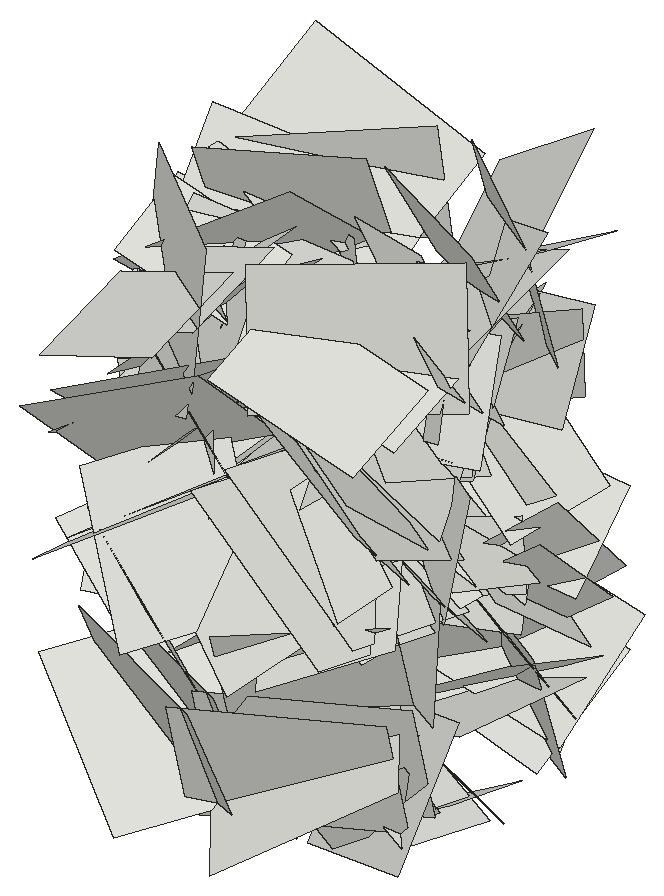
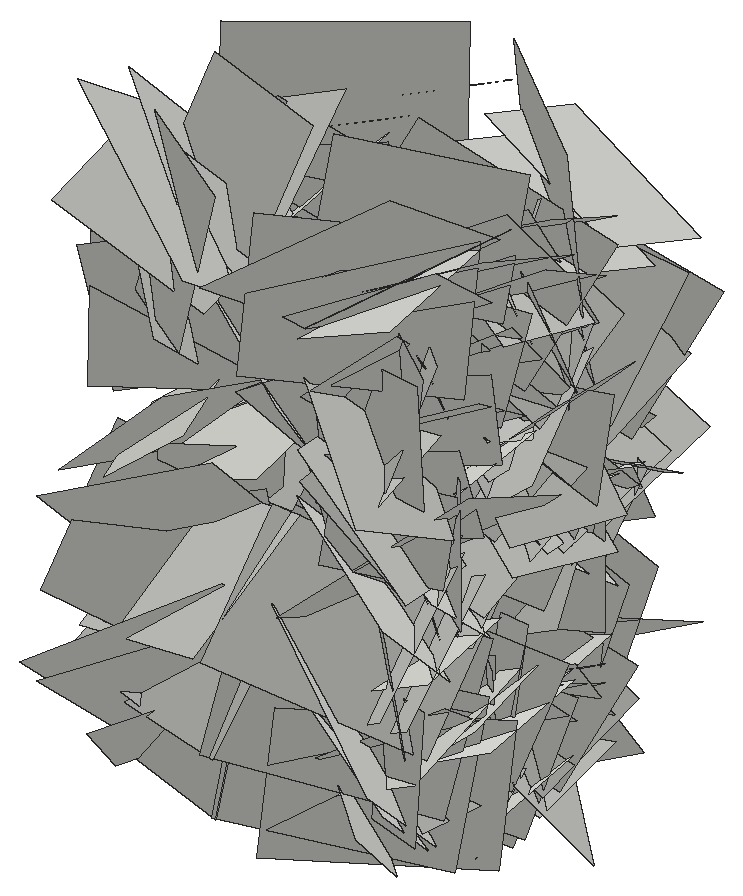
# SketchUp Ruby script. Lengths in inches.
U = 1.inch
M = Sketchup.active_model
def pt(a) = Geom::Point3d.new(a.map { |v| v * U })
def face(e, loops, mat)
  f = e.add_face(loops[0].map { |a| pt(a) })
  loops[1..].each { |l| e.add_face(l.map { |a| pt(a) }).erase! }
  f.material = f.back_material = mat if mat
  f
end
# faces: each face lists its corners as indices into pts; further lists are holes
def faces(e, pts, list, mat = nil) = list.each { |f| face(e, (f[0].is_a?(Array) ? f : [f]).map { |l| l.map { |i| pts[i] } }, mat) }
# xy, xz, yz: faces in a plane at the given z, y or x. An outline is a flat list of corners, or four numbers for a rectangle; further outlines are holes
def ring(l) = l.size == 4 ? [[l[0], l[1]], [l[2], l[1]], [l[2], l[3]], [l[0], l[3]]] : l.each_slice(2).to_a
def flat(e, list, mat, &to3) = list.each { |f| face(e, (f[0].is_a?(Array) ? f : [f]).map { |l| ring(l).map { |u, v| to3.(u, v) } }, mat) }
def xy(e, z, list, mat = nil) = flat(e, list, mat) { |x, y| [x, y, z] }
def xz(e, y, list, mat = nil) = flat(e, list, mat) { |x, z| [x, y, z] }
def yz(e, x, list, mat = nil) = flat(e, list, mat) { |y, z| [x, y, z] }
def lines(e, pts, list) = list.each { |a, b| e.add_line(pt(pts[a]), pt(pts[b])) }
# prism: a flat outline (further loops are holes) pulled along v
def prism(e, loops, v, mat = nil)
  f = face(e, loops, mat); d = Geom::Vector3d.new(v.map { |x| x * U })
  f.pushpull(f.normal.samedirection?(d) ? d.length : -d.length)
end
def box(e, o, s, mat = nil) = prism(e, [[o, [o[0] + s[0], o[1], o[2]], [o[0] + s[0], o[1] + s[1], o[2]], [o[0], o[1] + s[1], o[2]]]], [0, 0, s[2]], mat)
def at(x, y, z, deg = 0) = Geom::Transformation.translation(pt([x, y, z])) * Geom::Transformation.rotation(ORIGIN, Z_AXIS, deg.degrees)
def axes(o, x, y, z) = Geom::Transformation.new([*x, 0, *y, 0, *z, 0, *pt(o).to_a, 1])
def part(name) = M.definitions.add(name)
# library, detail: a bought-in or finely detailed component or shape, given as its bounding box
def library(name, o, s) = part(name).tap { |d| box(d.entities, o, s) }
def detail(e, o, s) = box(e.add_group.entities, o, s)
def put(e, d, t, mat = nil) = e.add_instance(d, t).tap { |i| i.material = mat if mat }
def group(e, t, mat = nil) = e.add_group.tap { |g| g.transformation = t; g.material = mat if mat }.entities
root = M.entities
c1 = part("Component\#6")
p = [[0.01,0,0],[0,3.24,4.54],[4.32,3.24,4.54],[4.33,0,0]]
faces(c1.entities,p,[[0,1,2,3]])
put(root,c1,axes([410.71,132.67,11.61],[-0.16439,-1.14375,-0.17253],[-0.24163,-0.14044,1.13591],[1.20204,-0.18465,0.20475]))
put(root,c1,axes([414.68,132.67,11.61],[0.16439,-1.14375,-0.17253],[0.24163,-0.14044,1.13591],[-1.20204,-0.18465,0.20475]))
put(root,c1,axes([410.71,126.24,11.02],[0.17433,0.41563,0.4957],[0.04437,0.50356,-0.43611],[0.68427,-0.13854,-0.09801]))
put(root,c1,axes([414.68,133.51,8.98],[0.15319,0.47062,-0.90401],[0.09722,-0.91536,-0.46187],[-1.07594,-0.0157,-0.17044]))
put(root,c1,axes([410.71,136.01,11.51],[0.06598,-0.27091,0.62957],[0.16839,0.62065,0.25136],[0.70672,-0.12259,-0.11867]))
put(root,c1,axes([410.71,130.2,1.79],[-0.1042,-0.77086,0.73803],[-0.17604,0.74317,0.75412],[1.11745,0.04519,0.18762]))
put(root,c1,axes([410.71,137.27,19.36],[-0.1763,0.15017,-0.9005],[0.15684,-0.89878,-0.17721],[0.95491,0.17535,-0.13715]))
put(root,c1,axes([414.68,136.42,13.64],[-0.14309,-0.55174,0.41683],[0.03038,0.41987,0.56505],[-0.73236,0.12522,-0.058]))
put(root,c1,axes([414.68,135.65,2.32],[0.1935,-1.06071,0.09437],[0.13048,0.11613,1.0671],[-1.12123,-0.16954,0.14047]))
put(root,c1,axes([410.71,132.96,18.89],[-0.10145,-0.91774,-0.17179],[0.02227,-0.17476,0.92192],[0.98945,-0.09016,-0.03837]))
put(root,c1,axes([410.71,133.07,14.74],[-0.12706,0.28525,0.91315],[0.02767,0.92092,-0.28425],[1.01369,0.01061,0.12222]))
put(root,c1,axes([410.71,135.14,15.06],[-0.15738,0.18416,-1.10832],[-0.16264,-1.1108,-0.16402],[1.17977,-0.12857,-0.17046]))
put(root,c1,axes([414.68,130.01,4.69],[-0.05447,0.12092,0.77662],[0.06993,0.77619,-0.11649],[-0.83019,0.05744,-0.06077]))
put(root,c1,axes([410.71,131.35,15.19],[0.02447,0.82058,-0.14823],[0.01236,-0.14859,-0.82075],[0.8838,-0.02064,0.01558]))
put(root,c1,axes([410.71,133.58,20.74],[-0.06025,0.71815,0.57437],[-0.00066,0.57544,-0.71955],[0.97476,0.04478,0.03501]))
put(root,c1,axes([410.71,133.14,16.06],[-0.03738,-0.31853,0.81486],[0.04959,0.81367,0.32009],[0.92608,-0.05642,0.01575]))
put(root,c1,axes([414.68,137.37,4.77],[0.01509,-0.67708,-0.46908],[0.05072,-0.46768,0.67651],[-0.87164,-0.03894,0.03124]))
put(root,c1,axes([410.71,128.53,16.93],[-0.30517,1.08519,-0.55956],[-0.1011,-0.59314,-1.10124],[1.29027,0.21019,-0.21864]))
put(root,c1,axes([410.71,127.92,4.7],[0.092,0.70183,0.2556],[0.07294,0.24871,-0.70628],[0.78837,-0.10491,0.03552]))
put(root,c1,axes([410.71,125.93,11.7],[0.16945,0.67455,-0.05214],[0.09647,-0.07453,-0.68517],[0.71064,-0.15073,0.10544]))
put(root,c1,axes([414.68,136.82,15.87],[0.16772,-0.74319,-0.48228],[-0.03783,-0.49486,0.75087],[-0.93836,-0.11289,-0.11647]))
put(root,c1,axes([414.68,131.86,3.01],[-0.01467,-0.55248,-0.51034],[0.00827,-0.51051,0.55244],[-0.7972,0.00487,0.01512]))
put(root,c1,axes([414.68,125.86,8.82],[-0.02658,0.53015,0.39509],[-0.11889,0.38623,-0.52538],[-0.69069,-0.08688,0.07523]))
put(root,c1,axes([410.71,127.95,5.4],[0.05879,0.74539,0.22064],[0.10629,0.21249,-0.74307],[0.81711,-0.08127,0.08079]))
put(root,c1,axes([414.68,131.99,-0.9375],[-0.0225,-0.54484,0.50649],[0.02225,0.50605,0.54525],[-0.78821,0.02984,0.00093]))
put(root,c1,axes([410.71,136.53,11.26],[-0.01536,-0.64622,-0.54667],[0.11065,-0.54394,0.64022],[0.89037,0.05645,-0.089]))
put(root,c1,axes([414.68,133.96,6.46],[0.0893,0.11056,0.97068],[0.19494,0.95507,-0.12474],[-1.01706,0.19277,0.06132]))
put(root,c1,axes([414.68,133.42,16.97],[0.14677,0.94615,0.46149],[0.22557,0.4307,-0.94687],[-1.09283,0.21597,-0.13346]))
put(root,c1,axes([410.71,127.34,21.1],[-0.03089,0.79811,0.32897],[0.11706,0.3299,-0.79059],[0.90753,-0.01539,0.11317]))
put(root,c1,axes([410.71,127.86,19.19],[-0.25173,1.01088,0.57921],[-0.04385,0.58343,-1.03521],[1.23418,0.22691,0.08136]))
put(root,c1,axes([414.68,129.8,15.91],[-0.05085,-0.71724,0.33006],[0.13843,0.31891,0.71198],[-0.82538,0.09767,0.09907]))
put(root,c1,axes([414.68,128.34,18.92],[-0.04874,0.38349,0.62334],[0.06251,0.62448,-0.37984],[-0.77325,0.02631,-0.07]))
put(root,c1,axes([410.71,132.55,10.48],[-0.11298,-1.07137,-0.22101],[-0.09706,-0.21254,1.07447],[1.1555,-0.12261,0.06864]))
put(root,c1,axes([414.68,129.18,10.77],[-0.08644,0.04023,-0.60323],[-0.06997,-0.60565,-0.03147],[-0.63702,0.06107,0.08531]))
put(root,c1,axes([410.71,132.5,3.06],[-0.12033,-0.77552,-0.96336],[-0.26418,-0.93322,0.78062],[1.28404,-0.26468,0.07033]))
put(root,c1,axes([414.68,129.23,5.41],[0.17398,-0.60139,0.60701],[-0.02487,0.6147,0.61536],[-0.9054,-0.13245,0.09973]))
put(root,c1,axes([414.68,130.03,2.94],[0.11679,-0.3481,0.76621],[0.04914,0.77408,0.34502],[-0.89071,-0.00294,0.1195]))
put(root,c1,axes([410.71,136.93,7.59],[-0.11136,0.24127,-0.97313],[0.07388,-0.97433,-0.24909],[1.06018,0.09324,-0.08486]))
put(root,c1,axes([414.68,133.88,6.93],[0.12434,-0.60409,0.41763],[-0.12699,0.40152,0.61444],[-0.76804,-0.16419,-0.03398]))
put(root,c1,axes([410.71,131.05,1.96],[-0.03915,-1.05631,0.36623],[-0.17317,0.36759,1.04378],[1.17236,0.01903,0.16641]))
put(root,c1,axes([410.71,133.1,9.3125],[-0.02086,0.87239,-0.16813],[0.14049,-0.16341,-0.8634],[0.93122,0.04419,0.12649]))
put(root,c1,axes([410.71,127.6,6.32],[0.09105,0.77875,-0.27248],[0.08108,-0.28029,-0.77696],[0.87078,-0.05533,0.10084]))
put(root,c1,axes([410.71,133.96,12.5],[0.03937,0.24323,0.81298],[0.12274,0.80469,-0.24604],[0.89109,-0.12158,-0.00203]))
put(root,c1,axes([414.68,132.63,6.14],[0.10731,0.87556,-0.00554],[0.12201,-0.01884,-0.87366],[-0.92006,0.09962,-0.1165]))
put(root,c1,axes([414.68,129.41,10.95],[0.18775,-0.48629,-0.69123],[-0.00245,-0.70652,0.49646],[-0.89586,-0.09998,-0.14623]))
put(root,c1,axes([410.71,129.45,15.69],[-0.00555,0.72683,0.86308],[-0.19522,0.85097,-0.71774],[1.18002,0.1442,-0.11468]))
put(root,c1,axes([414.68,129.84,16.13],[-0.05288,0.68465,0.04631],[0.09068,0.05228,-0.68068],[-0.72171,-0.04359,-0.08892]))
put(root,c1,axes([414.68,133.3125,17.59],[-0.01529,0.27468,0.5349],[-0.08187,0.52978,-0.27413],[-0.6321,-0.07526,0.02257]))
put(root,c1,axes([410.71,132.6,22.9],[0.05818,0.99288,0.05669],[-0.07779,0.06066,-0.99145],[1.05129,-0.05046,-0.07649]))
put(root,c1,axes([410.71,129.28,18.375],[0.15104,-0.37703,-0.77667],[-0.00911,-0.78776,0.38083],[0.9151,0.05438,0.13199]))
put(root,c1,axes([410.71,130.125,12.36],[-0.14413,1.23778,0.56401],[-0.30073,0.52855,-1.22835],[1.41013,0.23923,-0.20431]))
put(root,c1,axes([414.68,130.57,14.69],[0.08088,0.56373,-0.36339],[-0.06437,-0.35843,-0.56878],[-0.70803,0.09698,0.0102]))
put(root,c1,axes([414.68,131.53,3.64],[0.03356,0.34972,-0.55611],[-0.01458,-0.55628,-0.35061],[-0.69619,0.02851,-0.01946]))
put(root,c1,axes([410.71,133.79,15.82],[0.11741,-0.82822,-0.37202],[0.00882,-0.37384,0.83474],[0.96237,0.10447,0.03774]))
put(root,c1,axes([414.68,132.11,13.83],[0.12823,-0.67114,-0.46171],[0.10246,-0.45164,0.68184],[-0.85739,-0.15435,0.01243]))
put(root,c1,axes([410.71,128.52,17.74],[0.08604,0.43028,-0.81229],[0.04293,-0.81633,-0.42838],[0.97342,-0.00203,0.0907]))
put(root,c1,axes([414.68,134.57,7.51],[0.06425,-0.0713,-0.65597],[-0.02618,-0.65852,0.06929],[-0.69893,0.01811,-0.0629]))
put(root,c1,axes([410.71,133.2,0.29],[-0.16868,0.00753,1.30134],[-0.16064,1.302,-0.02607],[1.37005,0.15359,0.15716]))
put(root,c1,axes([414.68,127.28,0.51],[0.04452,-0.40985,0.5808],[0.07759,0.58122,0.40485],[-0.7495,0.03582,0.07641]))
put(root,c1,axes([410.71,129.68,16.21],[0.16446,-0.17941,-0.82447],[0.07006,-0.83314,0.19373],[0.89165,0.09856,0.13685]))
put(root,c1,axes([414.68,134.26,15.51],[0.13639,0.72841,-0.25059],[0.07067,-0.26364,-0.7321],[-0.81346,0.09922,-0.10562]))
put(root,c1,axes([410.71,128.87,2.92],[0.01411,0.95221,-0.19006],[0.11482,-0.19035,-0.94606],[1.02282,0.00823,0.10882]))
put(root,c1,axes([410.71,138.97,11.375],[-0.02639,-0.72989,-0.72722],[0.07911,-0.7268,0.72691],[1.08928,0.0351,-0.07041]))
put(root,c1,axes([410.71,131.74,20.5625],[-0.11289,-0.41624,-1.03402],[0.06809,-1.03929,0.41174],[1.17957,0.02016,-0.12272]))
put(root,c1,axes([414.68,131.9,7.66],[0.03371,0.19161,0.61883],[0.06203,0.6162,-0.1938],[-0.68388,0.06533,0.01292]))
put(root,c1,axes([410.71,134.95,12.42],[0.03363,0.92541,-1.00089],[-0.39451,-0.95725,-0.89685],[1.39004,-0.29406,-0.23032]))
put(root,c1,axes([414.68,131.8,8.64],[0.08497,0.05507,0.67491],[0.04101,0.67814,-0.05993],[-0.71661,0.04534,0.0766]))
put(root,c1,axes([410.71,137.87,11.82],[0.23548,-0.98581,-0.19043],[-0.17104,-0.22756,0.98976],[1.05044,0.18394,0.20385]))
put(root,c1,axes([410.71,129.625,19.87],[-0.14331,0.9196,0.97349],[-0.15794,0.96203,-0.92947],[1.41069,0.20113,-0.00516]))
put(root,c1,axes([410.71,130.99,8.6],[0.04494,-0.64922,0.68663],[0.20873,0.6783,0.62918],[0.97967,-0.11474,-0.16555]))
put(root,c1,axes([410.71,133.91,11.1875],[-0.02059,0.92356,-0.8814],[-0.20413,-0.87353,-0.91107],[1.33776,-0.11908,-0.15259]))
put(root,c1,axes([410.71,128.56,10.3125],[-0.23413,0.04823,1.24691],[0.1221,1.26168,-0.02839],[1.31707,-0.10839,0.22429]))
put(root,c1,axes([410.71,131.94,16.85],[-0.08825,-0.96476,0.81898],[-0.08011,0.82307,0.9619],[1.33903,-0.01434,0.11152]))
put(root,c1,axes([410.71,131.18,15.16],[0.15294,-1.16278,0.39158],[-0.28955,0.35393,1.15166],[1.26792,0.22109,0.21577]))
put(root,c1,axes([414.68,134.77,2.57],[0.05447,0.40704,0.46107],[0.08155,0.45478,-0.41007],[-0.64681,0.09162,-0.01288]))
put(root,c1,axes([410.71,134.14,22.88],[0.03825,0.99518,-0.25742],[0.13842,-0.25993,-0.98657],[1.08078,-0.00193,0.13547]))
put(root,c1,axes([410,124.93,11.12],[0.54058,0.75668,0.32998],[0.30141,0.20311,-0.90522],[0.82148,-0.57246,0.11499]))
put(root,c1,axes([410.71,127.92,6.47],[-0.03611,0.05394,1.13531],[0.09971,1.13206,-0.05096],[1.20066,-0.09239,0.03838]))
put(root,c1,axes([414.68,138.1,17.99],[0.00934,-0.49027,-0.41508],[0.1892,-0.3969,0.47259],[-0.65411,-0.1218,0.13076]))
put(root,c1,axes([410.71,127.69,20.12],[-0.02742,-1.01137,-0.35231],[0.21232,-0.35076,0.99222],[1.1152,0.04191,-0.19757]))
put(root,c1,axes([410.71,130,20.12],[-0.02742,-1.01137,-0.35231],[0.21232,-0.35076,0.99222],[1.1152,0.04191,-0.19757]))
put(root,c1,axes([414.68,129.35,18.22],[0.07955,-0.40219,0.442],[0.06566,0.44831,0.39741],[-0.63004,-0.00406,0.09723]))
put(root,c1,axes([410.71,129.81,24.32],[-0.08615,-0.07511,-1.33483],[-0.12267,-1.33188,0.08199],[1.41184,-0.12031,-0.07433]))
put(root,c1,axes([410.71,131.16,1.32],[0.11103,-1.00768,0.14491],[0.13016,0.15712,1.00381],[1.07125,0.08535,-0.13699]))
put(root,c1,axes([410.71,136.29,19.65],[0.239,0.33681,-1.04778],[-0.13934,-1.05364,-0.36698],[1.15826,-0.19625,0.17205]))
put(root,c1,axes([410.71,129.42,5.47],[-0.26825,1.30607,0.06413],[0.25565,0.11082,-1.30519],[1.36232,0.23638,0.25756]))
put(root,c1,axes([410.71,126.61,12.8],[-0.1414,-0.87971,0.87765],[0.19082,0.8597,0.88908],[1.30331,-0.22132,-0.03495]))
put(root,c1,axes([410.71,133.96,9.66],[0.06967,-1.04066,0.34132],[0.1454,0.34706,1.03175],[1.15177,0.01914,-0.15089]))
put(root,c1,axes([410.71,134.94,17.85],[0.08672,-0.29938,1.1859],[-0.04442,1.18717,0.30259],[1.29573,0.06074,-0.069]))
put(root,c1,axes([410.71,129.48,20.64],[-0.14207,1.22324,0.51937],[0.11373,0.53026,-1.2212],[1.40407,0.08082,0.15147]))
put(root,c1,axes([410.71,129.66,12.47],[-0.1081,-1.2535,0.58167],[-0.00417,0.58351,1.25678],[1.46479,-0.09085,0.0465]))
put(root,c1,axes([410.71,125.82,11.42],[0.20547,0.4933,-0.99975],[0.03886,-1.01702,-0.49472],[1.18108,-0.05236,0.1902]))
put(root,c1,axes([410.71,131.95,0.87],[0.07095,-0.70744,0.83659],[0.30432,0.82019,0.6706],[1.12076,-0.17792,-0.23504]))
put(root,c1,axes([410.71,139.8125,5.82],[0.12038,-0.94885,-0.86303],[-0.08352,-0.86993,0.94607],[1.35702,0.03063,0.13479]))
put(root,c1,axes([410.71,133.04,19.75],[0.14526,-0.49923,0.95494],[0.24012,0.95446,0.46647],[1.11669,-0.1403,-0.22453]))
put(root,c1,axes([410.71,128.24,17.68],[0.22785,0.52614,1.07761],[-0.06777,1.09826,-0.52347],[1.26934,-0.03581,-0.22138]))
put(root,c1,axes([410.71,133.15,22.79],[0.15509,1.06813,0.73269],[-0.10614,0.74447,-1.06531],[1.36888,-0.06329,-0.16562]))
put(root,c1,axes([410.71,132.12,7.08],[-0.00585,1.22451,-0.43101],[0.11167,-0.42917,-1.22063],[1.3715,0.04016,0.09755]))
put(root,c1,axes([410.71,125.99,1.35],[0.00241,0.79041,1.08039],[0.06651,1.07914,-0.78963],[1.41741,-0.05198,0.03522]))
put(root,c1,axes([410.71,127.67,13.74],[0.06329,-0.97705,0.81505],[0.12838,0.8166,0.97005],[1.34259,-0.03203,-0.13118]))
put(root,c1,axes([410.71,137,19.49],[0.23927,-0.1296,-1.18474],[0.04055,-1.20439,0.13904],[1.26266,0.06324,0.22004]))
put(root,c1,axes([410.71,135.39,1.18],[0.01455,-0.40823,1.27358],[0.1801,1.26386,0.40328],[1.40617,-0.15765,-0.06483]))
put(root,c1,axes([410.71,128.0625,10.23],[0.10909,-1.3698,0.20566],[-0.00727,0.20572,1.37363],[1.46824,0.1028,-0.00848]))
put(root,c1,axes([410.71,129.98,10.23],[0.10909,-1.3698,0.20566],[-0.00727,0.20572,1.37363],[1.46824,0.1028,-0.00848]))
put(root,c1,axes([410.71,138.98,4.78],[0.22268,-0.9196,-0.8307],[0.07298,-0.83259,0.9391],[1.31157,0.20246,0.08879]))
put(root,c1,axes([409.54,124.5,5.79],[0.83668,1.07369,0.2523],[0.21003,0.16716,-1.33127],[1.15009,-0.81162,0.05958]))
put(root,c1,axes([410.71,130.78,10.54],[0.24762,-1.26357,-0.1726],[-0.00687,-0.17664,1.28442],[1.3518,0.23056,0.03815]))
put(root,c1,axes([410.71,136.82,5.83],[0.1656,-1.02965,0.80161],[0.14776,0.81588,1.02082],[1.37528,0.03632,-0.2062]))
put(root,c1,axes([410.71,130.15,15.41],[0.24379,0.89731,1.03665],[0.02149,1.04879,-0.91232],[1.45316,-0.16605,-0.16042]))
put(root,c1,axes([410.71,135.96,3.29],[0.1622,-0.76384,1.11136],[0.23079,1.11781,0.7383],[1.4107,-0.09505,-0.24857]))
put(root,c1,axes([410.71,125.3125,7.6875],[0.15543,0.49215,-1.26812],[0.29157,-1.25984,-0.45713],[1.41209,0.20597,0.23397]))
put(root,c1,axes([410.71,126.76,7.6875],[0.15543,0.49215,-1.26812],[0.29157,-1.25984,-0.45713],[1.41209,0.20597,0.23397]))
put(root,c1,axes([410.61,125.5,13.2],[1.07209,0.56535,0.5401],[0.40295,0.41611,-1.14744],[0.72423,-1.06841,-0.1611]))
put(root,c1,axes([424.6,125.5,13.2],[-1.07209,0.56535,0.5401],[-0.40295,0.41611,-1.14744],[-0.72423,-1.06841,-0.1611]))
put(root,c1,axes([424.49,125.3125,7.6875],[-0.15543,0.49215,-1.26812],[-0.29157,-1.25984,-0.45713],[-1.41209,0.20597,0.23397]))
put(root,c1,axes([424.49,126.76,7.6875],[-0.15543,0.49215,-1.26812],[-0.29157,-1.25984,-0.45713],[-1.41209,0.20597,0.23397]))
put(root,c1,axes([424.49,135.96,3.29],[-0.1622,-0.76384,1.11136],[-0.23079,1.11781,0.7383],[-1.4107,-0.09505,-0.24857]))
put(root,c1,axes([424.49,130.15,15.41],[-0.24379,0.89731,1.03665],[-0.02149,1.04879,-0.91232],[-1.45316,-0.16605,-0.16042]))
put(root,c1,axes([424.49,136.82,5.83],[-0.1656,-1.02965,0.80161],[-0.14776,0.81588,1.02082],[-1.37528,0.03632,-0.2062]))
put(root,c1,axes([424.49,130.78,10.54],[-0.24762,-1.26357,-0.1726],[0.00687,-0.17664,1.28442],[-1.3518,0.23056,0.03815]))
put(root,c1,axes([425.66,124.5,5.79],[-0.83668,1.07369,0.2523],[-0.21003,0.16716,-1.33127],[-1.15009,-0.81162,0.05958]))
put(root,c1,axes([424.49,138.98,4.78],[-0.22268,-0.9196,-0.8307],[-0.07298,-0.83259,0.9391],[-1.31157,0.20246,0.08879]))
put(root,c1,axes([424.49,128.0625,10.23],[-0.10909,-1.3698,0.20566],[0.00727,0.20572,1.37363],[-1.46824,0.1028,-0.00848]))
put(root,c1,axes([424.49,129.98,10.23],[-0.10909,-1.3698,0.20566],[0.00727,0.20572,1.37363],[-1.46824,0.1028,-0.00848]))
put(root,c1,axes([424.49,135.39,1.18],[-0.01455,-0.40823,1.27358],[-0.1801,1.26386,0.40328],[-1.40617,-0.15765,-0.06483]))
put(root,c1,axes([424.49,137,19.49],[-0.23927,-0.1296,-1.18474],[-0.04055,-1.20439,0.13904],[-1.26266,0.06324,0.22004]))
put(root,c1,axes([424.49,127.67,13.74],[-0.06329,-0.97705,0.81505],[-0.12838,0.8166,0.97005],[-1.34259,-0.03203,-0.13118]))
put(root,c1,axes([424.49,125.99,1.35],[-0.00241,0.79041,1.08039],[-0.06651,1.07914,-0.78963],[-1.41741,-0.05198,0.03522]))
put(root,c1,axes([424.49,132.12,7.08],[0.00585,1.22451,-0.43101],[-0.11167,-0.42917,-1.22063],[-1.3715,0.04016,0.09755]))
put(root,c1,axes([424.49,133.15,22.79],[-0.15509,1.06813,0.73269],[0.10614,0.74447,-1.06531],[-1.36888,-0.06329,-0.16562]))
put(root,c1,axes([424.49,128.24,17.68],[-0.22785,0.52614,1.07761],[0.06777,1.09826,-0.52347],[-1.26934,-0.03581,-0.22138]))
put(root,c1,axes([424.49,133.04,19.75],[-0.14526,-0.49923,0.95494],[-0.24012,0.95446,0.46647],[-1.11669,-0.1403,-0.22453]))
put(root,c1,axes([424.49,139.8125,5.82],[-0.12038,-0.94885,-0.86303],[0.08352,-0.86993,0.94607],[-1.35702,0.03063,0.13479]))
put(root,c1,axes([424.49,131.95,0.87],[-0.07095,-0.70744,0.83659],[-0.30432,0.82019,0.6706],[-1.12076,-0.17792,-0.23504]))
put(root,c1,axes([424.49,125.82,11.42],[-0.20547,0.4933,-0.99975],[-0.03886,-1.01702,-0.49472],[-1.18108,-0.05236,0.1902]))
put(root,c1,axes([424.49,129.66,12.47],[0.1081,-1.2535,0.58167],[0.00417,0.58351,1.25678],[-1.46479,-0.09085,0.0465]))
put(root,c1,axes([424.49,129.48,20.64],[0.14207,1.22324,0.51937],[-0.11373,0.53026,-1.2212],[-1.40407,0.08082,0.15147]))
put(root,c1,axes([424.49,134.94,17.85],[-0.08672,-0.29938,1.1859],[0.04442,1.18717,0.30259],[-1.29573,0.06074,-0.069]))
put(root,c1,axes([424.49,133.96,9.66],[-0.06967,-1.04066,0.34132],[-0.1454,0.34706,1.03175],[-1.15177,0.01914,-0.15089]))
put(root,c1,axes([424.49,126.61,12.8],[0.1414,-0.87971,0.87765],[-0.19082,0.8597,0.88908],[-1.30331,-0.22132,-0.03495]))
put(root,c1,axes([424.49,129.42,5.47],[0.26825,1.30607,0.06413],[-0.25565,0.11082,-1.30519],[-1.36232,0.23638,0.25756]))
put(root,c1,axes([424.49,136.29,19.65],[-0.239,0.33681,-1.04778],[0.13934,-1.05364,-0.36698],[-1.15826,-0.19625,0.17205]))
put(root,c1,axes([424.49,131.16,1.32],[-0.11103,-1.00768,0.14491],[-0.13016,0.15712,1.00381],[-1.07125,0.08535,-0.13699]))
put(root,c1,axes([424.49,129.81,24.32],[0.08615,-0.07511,-1.33483],[0.12267,-1.33188,0.08199],[-1.41184,-0.12031,-0.07433]))
put(root,c1,axes([420.52,129.35,18.22],[-0.07955,-0.40219,0.442],[-0.06566,0.44831,0.39741],[0.63004,-0.00406,0.09723]))
put(root,c1,axes([424.49,127.69,20.12],[0.02742,-1.01137,-0.35231],[-0.21232,-0.35076,0.99222],[-1.1152,0.04191,-0.19757]))
put(root,c1,axes([424.49,130,20.12],[0.02742,-1.01137,-0.35231],[-0.21232,-0.35076,0.99222],[-1.1152,0.04191,-0.19757]))
put(root,c1,axes([420.52,138.1,17.99],[-0.00934,-0.49027,-0.41508],[-0.1892,-0.3969,0.47259],[0.65411,-0.1218,0.13076]))
put(root,c1,axes([424.49,127.92,6.47],[0.03611,0.05394,1.13531],[-0.09971,1.13206,-0.05096],[-1.20066,-0.09239,0.03838]))
put(root,c1,axes([425.21,124.93,11.12],[-0.54058,0.75668,0.32998],[-0.30141,0.20311,-0.90522],[-0.82148,-0.57246,0.11499]))
put(root,c1,axes([424.49,134.14,22.88],[-0.03825,0.99518,-0.25742],[-0.13842,-0.25993,-0.98657],[-1.08078,-0.00193,0.13547]))
put(root,c1,axes([420.52,134.77,2.57],[-0.05447,0.40704,0.46107],[-0.08155,0.45478,-0.41007],[0.64681,0.09162,-0.01288]))
put(root,c1,axes([424.49,131.18,15.16],[-0.15294,-1.16278,0.39158],[0.28955,0.35393,1.15166],[-1.26792,0.22109,0.21577]))
put(root,c1,axes([424.49,131.94,16.85],[0.08825,-0.96476,0.81898],[0.08011,0.82307,0.9619],[-1.33903,-0.01434,0.11152]))
put(root,c1,axes([424.49,128.56,10.3125],[0.23413,0.04823,1.24691],[-0.1221,1.26168,-0.02839],[-1.31707,-0.10839,0.22429]))
put(root,c1,axes([424.49,133.91,11.1875],[0.02059,0.92356,-0.8814],[0.20413,-0.87353,-0.91107],[-1.33776,-0.11908,-0.15259]))
put(root,c1,axes([424.49,130.99,8.6],[-0.04494,-0.64922,0.68663],[-0.20873,0.6783,0.62918],[-0.97967,-0.11474,-0.16555]))
put(root,c1,axes([424.49,129.625,19.87],[0.14331,0.9196,0.97349],[0.15794,0.96203,-0.92947],[-1.41069,0.20113,-0.00516]))
put(root,c1,axes([424.49,137.87,11.82],[-0.23548,-0.98581,-0.19043],[0.17104,-0.22756,0.98976],[-1.05044,0.18394,0.20385]))
put(root,c1,axes([420.52,131.8,8.64],[-0.08497,0.05507,0.67491],[-0.04101,0.67814,-0.05993],[0.71661,0.04534,0.0766]))
put(root,c1,axes([424.49,134.95,12.42],[-0.03363,0.92541,-1.00089],[0.39451,-0.95725,-0.89685],[-1.39004,-0.29406,-0.23032]))
put(root,c1,axes([420.52,131.9,7.66],[-0.03371,0.19161,0.61883],[-0.06203,0.6162,-0.1938],[0.68388,0.06533,0.01292]))
put(root,c1,axes([424.49,131.74,20.5625],[0.11289,-0.41624,-1.03402],[-0.06809,-1.03929,0.41174],[-1.17957,0.02016,-0.12272]))
put(root,c1,axes([424.49,138.97,11.375],[0.02639,-0.72989,-0.72722],[-0.07911,-0.7268,0.72691],[-1.08928,0.0351,-0.07041]))
put(root,c1,axes([424.49,128.87,2.92],[-0.01411,0.95221,-0.19006],[-0.11482,-0.19035,-0.94606],[-1.02282,0.00823,0.10882]))
put(root,c1,axes([420.52,134.26,15.51],[-0.13639,0.72841,-0.25059],[-0.07067,-0.26364,-0.7321],[0.81346,0.09922,-0.10562]))
put(root,c1,axes([424.49,129.68,16.21],[-0.16446,-0.17941,-0.82447],[-0.07006,-0.83314,0.19373],[-0.89165,0.09856,0.13685]))
put(root,c1,axes([420.52,127.28,0.51],[-0.04452,-0.40985,0.5808],[-0.07759,0.58122,0.40485],[0.7495,0.03582,0.07641]))
